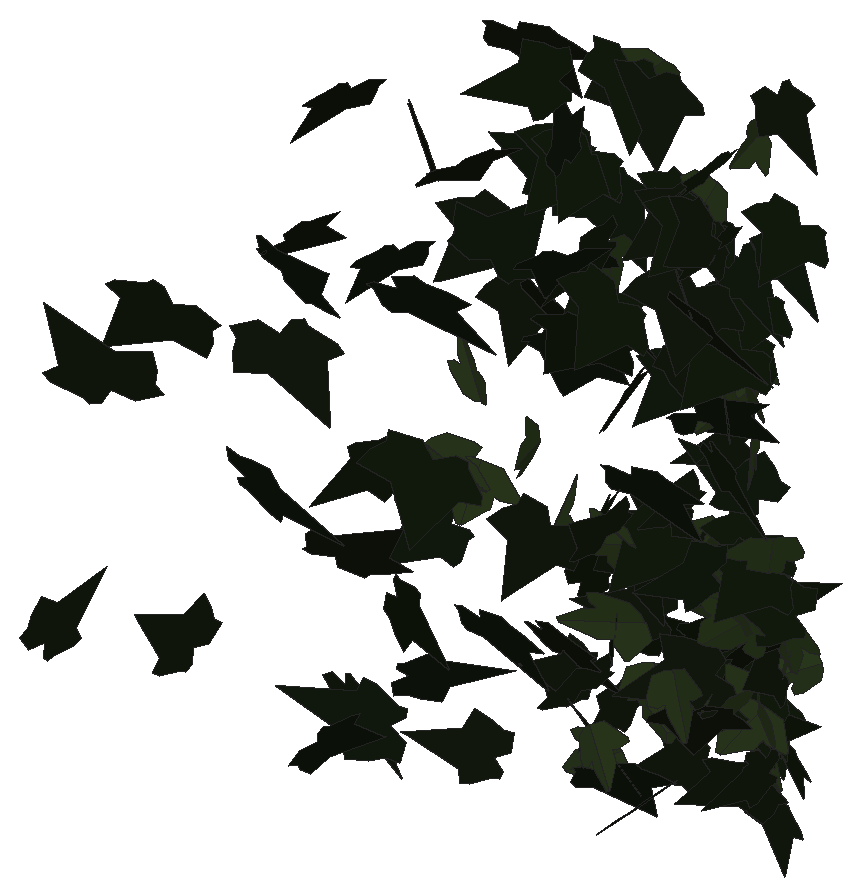
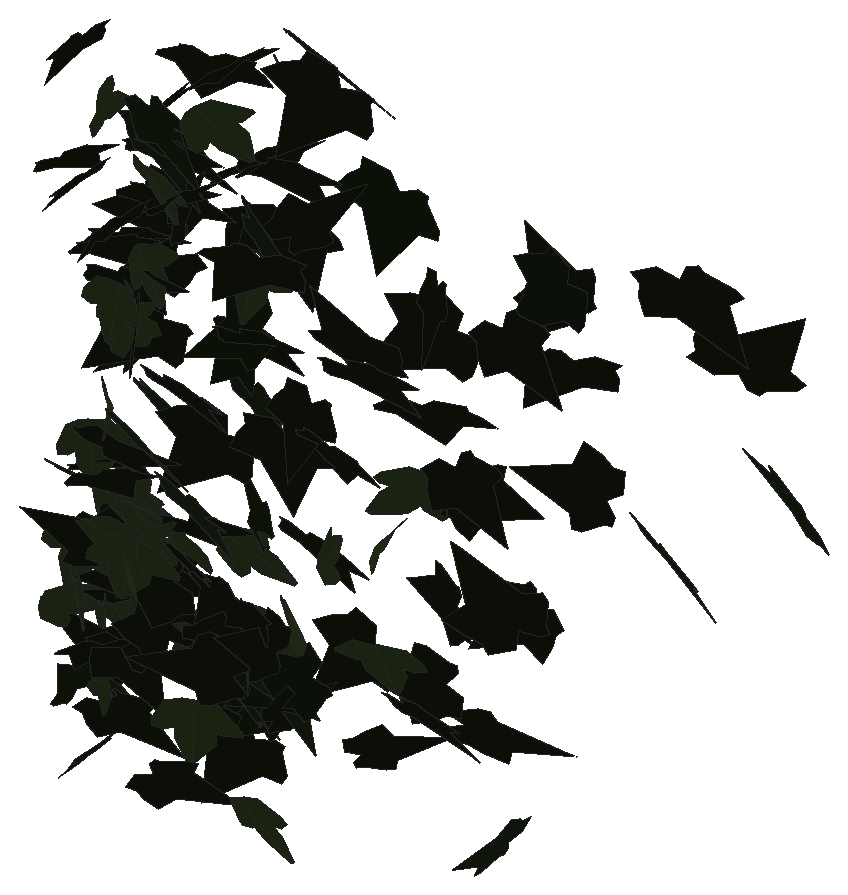
# SketchUp Ruby script. Lengths in inches.
U = 1.inch
M = Sketchup.active_model
def pt(a) = Geom::Point3d.new(a.map { |v| v * U })
def face(e, loops, mat)
  f = e.add_face(loops[0].map { |a| pt(a) })
  loops[1..].each { |l| e.add_face(l.map { |a| pt(a) }).erase! }
  f.material = f.back_material = mat if mat
  f
end
# faces: each face lists its corners as indices into pts; further lists are holes
def faces(e, pts, list, mat = nil) = list.each { |f| face(e, (f[0].is_a?(Array) ? f : [f]).map { |l| l.map { |i| pts[i] } }, mat) }
# xy, xz, yz: faces in a plane at the given z, y or x. An outline is a flat list of corners, or four numbers for a rectangle; further outlines are holes
def ring(l) = l.size == 4 ? [[l[0], l[1]], [l[2], l[1]], [l[2], l[3]], [l[0], l[3]]] : l.each_slice(2).to_a
def flat(e, list, mat, &to3) = list.each { |f| face(e, (f[0].is_a?(Array) ? f : [f]).map { |l| ring(l).map { |u, v| to3.(u, v) } }, mat) }
def xy(e, z, list, mat = nil) = flat(e, list, mat) { |x, y| [x, y, z] }
def xz(e, y, list, mat = nil) = flat(e, list, mat) { |x, z| [x, y, z] }
def yz(e, x, list, mat = nil) = flat(e, list, mat) { |y, z| [x, y, z] }
def lines(e, pts, list) = list.each { |a, b| e.add_line(pt(pts[a]), pt(pts[b])) }
# prism: a flat outline (further loops are holes) pulled along v
def prism(e, loops, v, mat = nil)
  f = face(e, loops, mat); d = Geom::Vector3d.new(v.map { |x| x * U })
  f.pushpull(f.normal.samedirection?(d) ? d.length : -d.length)
end
def box(e, o, s, mat = nil) = prism(e, [[o, [o[0] + s[0], o[1], o[2]], [o[0] + s[0], o[1] + s[1], o[2]], [o[0], o[1] + s[1], o[2]]]], [0, 0, s[2]], mat)
def at(x, y, z, deg = 0) = Geom::Transformation.translation(pt([x, y, z])) * Geom::Transformation.rotation(ORIGIN, Z_AXIS, deg.degrees)
def axes(o, x, y, z) = Geom::Transformation.new([*x, 0, *y, 0, *z, 0, *pt(o).to_a, 1])
def part(name) = M.definitions.add(name)
# library, detail: a bought-in or finely detailed component or shape, given as its bounding box
def library(name, o, s) = part(name).tap { |d| box(d.entities, o, s) }
def detail(e, o, s) = box(e.add_group.entities, o, s)
def put(e, d, t, mat = nil) = e.add_instance(d, t).tap { |i| i.material = mat if mat }
def group(e, t, mat = nil) = e.add_group.tap { |g| g.transformation = t; g.material = mat if mat }.entities
root = M.entities
M.materials.add("1026 AP 7946 SUNNY SIDE UP").color = [254, 231, 186]
M.materials.add("efeu1").color = [18, 25, 13]
M.materials.add("efeu2").color = [43, 57, 29]
c1 = part("ivyleaf_9")
p = [[1.54,2.16,1.25],[1.36,2.04,1.19],[-0.21,0.99,0.68],[-0.71,1.11,0.82],[-0.85,0.86,0.67],[-0.8,0.17,0.21],
  [-0.9,-0.01,0.1],[-0.67,-0.16,-0.02],[-0.08,-0.08,-0.05],[-0.03,-0.6,-0.4],[0.65,-0.88,-0.66],[0.83,-0.6,-0.49],
  [1.29,-0.42,-0.43],[1.8125,-0.07,-0.26],[1.21,0.44,0.15]]
faces(c1.entities,p,[[0,1,2,3,4,5,6,7,8,9,10,11,12,13,14]],"efeu1")
c2 = part("ivyleaf_10")
p = [[0,0.5,-0.03],[-0.0625,2.02,-0.43],[-0.19,2.01,-0.46],[-0.54,1.05,-0.29],[-0.52,0.625,-0.18],[-0.83,0.76,-0.28],
  [-1.16,0.64,-0.33],[-1.15,0.33,-0.24],[-0.77,-0.39,0.02],[-0.3,-0.51,0.16],[0.04,-0.48,0.23],[-0.02,2.01,-0.4375],
  [-0.06,2.01,-0.43],[0.04,-0.49,0.23],[0.67,-0.49,0.14],[1.38,0.36,-0.2],[1.375,0.51,-0.24],[0.81,0.65,-0.19],
  [0.62,0.59,-0.15],[0.6,1.09,-0.28],[0.5,1.23,-0.31]]
faces(c2.entities,p,[[0,1,2,3,4,5,6,7,8,9,10],[11,12,0,13,14,15,16,17,18,19,20]],"efeu2")
put(root,c1,axes([90.28,204.37,282.83],[-0.24358,0.38021,0.10952],[0.06838,-0.08884,0.43377],[0.66272,0.14891,-0.0045]),"1026 AP 7946 SUNNY SIDE UP")
put(root,c1,axes([90.01,206.08,285.99],[0.29721,0.05151,0.38408],[-0.60755,0.0827,0.17576],[-0.08959,-0.38992,0.08224]),"1026 AP 7946 SUNNY SIDE UP")
put(root,c1,axes([91.6,205.9,282.51],[-0.23197,0.30623,0.25862],[-0.19167,0.20953,-0.35575],[-0.6294,-0.17667,0.01302]),"1026 AP 7946 SUNNY SIDE UP")
put(root,c1,axes([90.74,206.5,287.33],[0.23481,0.09165,-0.38264],[-0.42428,-0.25925,-0.17776],[-0.46344,0.28377,-0.03114]),"1026 AP 7946 SUNNY SIDE UP")
put(root,c1,axes([93.29,206.64,281.26],[-0.08853,0.12697,-0.37628],[-0.15546,0.34144,0.15068],[0.61777,0.10412,-0.01601]),"1026 AP 7946 SUNNY SIDE UP")
put(root,c1,axes([91.22,207.6875,284.22],[0.40642,-0.15866,0.28639],[0.33268,-0.1885,-0.30774],[0.41385,0.30734,-0.03386]),"1026 AP 7946 SUNNY SIDE UP")
put(root,c1,axes([91.49,208.1,287.43],[0.57582,-0.10896,-0.15139],[0.2568,0.0199,0.37613],[-0.15728,-0.36642,0.05986]),"1026 AP 7946 SUNNY SIDE UP")
put(root,c1,axes([91.51,208.01,286.4375],[-0.16156,-0.27217,-0.28485],[0.1869,0.23904,-0.30471],[0.61412,-0.14435,0.0178]),"1026 AP 7946 SUNNY SIDE UP")
put(root,c1,axes([93.84,208.41,285.09],[-0.48199,-0.26527,-0.10385],[0.16958,0.02915,-0.41271],[0.44635,-0.29752,0.04466]),"1026 AP 7946 SUNNY SIDE UP")
put(root,c1,axes([91.42,208.27,287.83],[0.25122,0.26891,0.23765],[0.2212,0.17693,-0.32517],[-0.54497,0.19577,-0.02244]),"1026 AP 7946 SUNNY SIDE UP")
put(root,c1,axes([92.78,208.71,280.45],[-0.32348,-0.12983,-0.30399],[-0.39375,-0.16084,0.2446],[-0.35087,0.30019,0.00576]),"1026 AP 7946 SUNNY SIDE UP")
put(root,c1,axes([92.92,208.85,282.4],[0.09531,-0.09706,-0.3787],[0.61631,-0.02708,0.06952],[-0.07289,-0.35589,0.09263]),"1026 AP 7946 SUNNY SIDE UP")
put(root,c1,axes([96.6,209.03,288.3],[-0.25614,-0.32528,0.20811],[-0.10783,-0.18919,-0.38597],[0.63794,-0.16258,0.01832]),"1026 AP 7946 SUNNY SIDE UP")
put(root,c1,axes([92.53,209.01,284.44],[-0.10498,0.00796,-0.395],[0.14058,-0.36437,-0.02835],[-0.61067,-0.08525,0.06138]),"1026 AP 7946 SUNNY SIDE UP")
put(root,c1,axes([91.69,209.06,282.58],[0.59044,0.15415,-0.01146],[-0.0079,0.04169,0.40563],[0.26245,-0.34555,0.03798]),"1026 AP 7946 SUNNY SIDE UP")
put(root,c1,axes([96.49,208.91,284.66],[-0.14634,0.32567,0.15798],[-0.08423,0.13502,-0.35854],[-0.5981,-0.0987,0.01184]),"1026 AP 7946 SUNNY SIDE UP")
put(root,c1,axes([96.03,209.13,287.6],[0.27288,0.13159,-0.30791],[-0.34397,-0.20738,-0.22439],[-0.41571,0.25797,-0.01645]),"1026 AP 7946 SUNNY SIDE UP")
put(root,c1,axes([93.04,209.01,281.18],[0.18415,0.2178,-0.27133],[0.10731,0.25128,0.26078],[0.56076,-0.11961,0.0392]),"1026 AP 7946 SUNNY SIDE UP")
put(root,c1,axes([92.68,209.21,287.05],[0.6573,0.06501,0.09122],[0.15221,-0.02734,-0.41843],[-0.09756,0.39534,-0.03825]),"1026 AP 7946 SUNNY SIDE UP")
put(root,c1,axes([93.95,209.57,279.99],[-0.17113,-0.01295,0.33509],[-0.4862,-0.12982,-0.10626],[0.21613,-0.3023,0.02628]),"1026 AP 7946 SUNNY SIDE UP")
put(root,c2,axes([95.96,209.375,281.05],[0.07273,0.33107,0.01199],[0.01082,0.00611,-0.35726],[-0.56202,0.04296,-0.00533]),"1026 AP 7946 SUNNY SIDE UP")
put(root,c2,axes([97.1875,209.54,282.27],[0.4331,-0.08334,0.22855],[0.32153,-0.10601,-0.28667],[0.22204,0.31606,-0.03068]),"1026 AP 7946 SUNNY SIDE UP")
put(root,c1,axes([97.93,209.42,284.3125],[-0.45991,0.24915,0.02602],[-0.06086,-0.00798,-0.39284],[-0.42007,-0.27162,0.02842]),"1026 AP 7946 SUNNY SIDE UP")
put(root,c1,axes([96.71,209.28,280.24],[0.03469,0.37547,0.12003],[0.01979,0.10673,-0.40104],[-0.66257,0.02285,-0.0057]),"1026 AP 7946 SUNNY SIDE UP")
put(root,c2,axes([93.08,209.46,284.55],[-0.34261,-0.15364,-0.24766],[0.37491,0.08055,-0.26473],[0.28111,-0.29468,0.05122]),"1026 AP 7946 SUNNY SIDE UP")
put(root,c1,axes([95.04,209.62,291.03],[-0.54914,0.19561,0.07717],[-0.13967,-0.00261,-0.40199],[-0.32355,-0.33087,0.04256]),"1026 AP 7946 SUNNY SIDE UP")
put(root,c1,axes([97.42,210.05,289.23],[-0.17996,-0.19101,0.31705],[-0.17291,-0.28215,-0.23585],[0.5764,-0.14428,0.02824]),"1026 AP 7946 SUNNY SIDE UP")
put(root,c1,axes([95.3125,209.51,290.01],[0.00313,0.11265,0.39841],[-0.04172,0.36997,-0.11508],[-0.65633,-0.02298,0.00922]),"1026 AP 7946 SUNNY SIDE UP")
put(root,c1,axes([93.41,209.53,289.15],[0.2412,0.37899,0.09819],[0.03464,0.08499,-0.43199],[-0.65909,0.14316,0.01323]),"1026 AP 7946 SUNNY SIDE UP")
put(root,c1,axes([97.4375,209.69,281.83],[0.30649,0.26126,-0.1198],[-0.08848,-0.10398,-0.34105],[-0.47663,0.1873,-0.01372]),"1026 AP 7946 SUNNY SIDE UP")
put(root,c1,axes([93.67,209.79,281.92],[0.63362,-0.01268,-0.04615],[-0.0746,-0.03474,-0.39845],[0.01454,0.37411,-0.03329]),"1026 AP 7946 SUNNY SIDE UP")
put(root,c1,axes([95.12,209.8,288.19],[0.16397,0.32864,-0.15217],[-0.07703,-0.13927,-0.36864],[-0.60588,0.10665,0.00569]),"1026 AP 7946 SUNNY SIDE UP")
put(root,c1,axes([97.47,210.02,282.3],[-0.60196,0.06601,0.09509],[-0.15787,-0.02152,-0.38441],[-0.09963,-0.36472,0.03462]),"1026 AP 7946 SUNNY SIDE UP")
put(root,c1,axes([97.02,210.04,287.83],[0.44864,-0.16709,0.1738],[0.20653,-0.11421,-0.335],[0.34029,0.2896,-0.02582]),"1026 AP 7946 SUNNY SIDE UP")
put(root,c1,axes([91.03,210.08,279.79],[0.30427,-0.33021,-0.03507],[-0.01877,0.02637,-0.40186],[0.5623,0.17956,0.00556]),"1026 AP 7946 SUNNY SIDE UP")
put(root,c1,axes([94.49,210.16,283.52],[-0.59937,-0.03075,-0.15291],[0.24537,-0.02672,-0.37781],[0.03126,-0.37979,0.0336]),"1026 AP 7946 SUNNY SIDE UP")
put(root,c1,axes([97.04,210.21,288.15],[-0.48786,-0.2239,-0.13843],[0.20303,0.05137,-0.38788],[0.38636,-0.30972,0.02904]),"1026 AP 7946 SUNNY SIDE UP")
put(root,c1,axes([97.47,210.14,285.68],[0.36619,-0.27433,-0.05768],[-0.08023,0.02671,-0.3726],[0.4666,0.21989,-0.0188]),"1026 AP 7946 SUNNY SIDE UP")
put(root,c2,axes([97.75,210.35,282.01],[0.00476,-0.02498,0.3479],[0.03758,-0.32454,-0.03142],[0.55255,0.02229,-0.00086]),"1026 AP 7946 SUNNY SIDE UP")
put(root,c1,axes([95.03,210.39,289.49],[-0.24032,-0.31552,0.1567],[-0.05092,-0.1508,-0.3708],[0.59123,-0.14124,0.03176]),"1026 AP 7946 SUNNY SIDE UP")
put(root,c1,axes([97.69,210.35,287.37],[-0.50073,-0.20031,0.03423],[-0.01264,-0.05026,-0.38034],[0.34484,-0.29271,0.03576]),"1026 AP 7946 SUNNY SIDE UP")
put(root,c1,axes([95.42,210.24,288.3],[-0.4811,0.20682,-0.20993],[0.22752,-0.1516,-0.37554],[-0.43054,-0.31121,0.03613]),"1026 AP 7946 SUNNY SIDE UP")
put(root,c1,axes([97.09,210.4,289.13],[-0.41864,-0.21772,0.09656],[-0.08882,-0.0809,-0.3523],[0.39199,-0.25086,0.0233]),"1026 AP 7946 SUNNY SIDE UP")
put(root,c1,axes([97.49,210.0625,289],[-0.25637,0.33466,0.03547],[-0.06393,0.01448,-0.3917],[-0.5666,-0.15306,0.02814]),"1026 AP 7946 SUNNY SIDE UP")
put(root,c1,axes([95.04,210.2,280.72],[0.51109,-0.19488,-0.05836],[-0.09684,0.00728,-0.38295],[0.3284,0.30544,-0.0221]),"1026 AP 7946 SUNNY SIDE UP")
put(root,c2,axes([97.79,210.27,283.1],[-0.44981,0.00742,0.22798],[-0.35369,-0.07947,-0.27583],[0.07495,-0.33046,0.06657]),"1026 AP 7946 SUNNY SIDE UP")
put(root,c1,axes([95.92,209.97,286.09],[-0.16185,0.14812,-0.34149],[-0.33688,0.2526,0.19147],[0.49648,0.21969,0.0186]),"1026 AP 7946 SUNNY SIDE UP")
put(root,c1,axes([94.94,210.47,289.48],[-0.58601,-0.15376,-0.00557],[0.02315,-0.02278,-0.40391],[0.26004,-0.34447,0.0234]),"1026 AP 7946 SUNNY SIDE UP")
put(root,c1,axes([96.84,210.46,289.13],[-0.57945,-0.04375,0.01249],[-0.01272,-0.03722,-0.36693],[0.07606,-0.33953,0.03374]),"1026 AP 7946 SUNNY SIDE UP")
put(root,c2,axes([97.67,210.27,283.27],[-0.22751,0.04524,0.32245],[-0.50905,0.03417,-0.14817],[-0.08459,-0.32735,0.02439]),"1026 AP 7946 SUNNY SIDE UP")
put(root,c1,axes([95.09,210.41,283.54],[0.03299,0.24718,0.22068],[-0.07855,-0.19897,0.26145],[0.53715,-0.04428,0.02468]),"1026 AP 7946 SUNNY SIDE UP")
put(root,c1,axes([95.47,210.24,279.95],[0.48475,0.21422,0.00873],[0.03169,-0.01598,-0.38153],[-0.36237,0.28516,-0.02169]),"1026 AP 7946 SUNNY SIDE UP")
put(root,c1,axes([97.87,210.68,283.78],[-0.38029,-0.22783,0.12324],[-0.03763,-0.13899,-0.33404],[0.43398,-0.21169,0.07903]),"1026 AP 7946 SUNNY SIDE UP")
put(root,c1,axes([96.72,210.39,287.94],[0.06571,-0.26019,0.28328],[0.01202,0.26989,0.2832],[-0.63396,-0.02185,0.03473]),"1026 AP 7946 SUNNY SIDE UP")
put(root,c1,axes([95.52,210.66,290.96],[-0.09479,-0.38255,0.04381],[-0.01928,-0.04473,-0.41449],[0.65377,-0.05678,-0.00587]),"1026 AP 7946 SUNNY SIDE UP")
put(root,c1,axes([95.95,210.5625,290.9],[-0.38038,-0.23962,-0.19924],[0.2509,0.1114,-0.3484],[0.44607,-0.26699,0.02607]),"1026 AP 7946 SUNNY SIDE UP")
put(root,c1,axes([95.9,210.33,284.73],[0.636,0.07083,-0.02131],[-0.02333,-0.03897,-0.40696],[-0.12313,0.37321,-0.033]),"1026 AP 7946 SUNNY SIDE UP")
put(root,c1,axes([96.9,210.23,287.22],[0.12884,-0.06857,-0.39529],[-0.0414,0.37412,-0.07472],[0.63466,0.03832,0.07538]),"1026 AP 7946 SUNNY SIDE UP")
put(root,c2,axes([97.84,210.52,281.57],[0.53443,-0.00012,-0.12716],[-0.20044,-0.03686,-0.33553],[-0.0219,0.33446,-0.0323]),"1026 AP 7946 SUNNY SIDE UP")
put(root,c1,axes([95.51,210.59,280.94],[-0.42379,0.10851,-0.15282],[0.19254,-0.09703,-0.28982],[-0.23822,-0.27146,0.03763]),"1026 AP 7946 SUNNY SIDE UP")
put(root,c1,axes([93.85,210.36,291.03],[0.64688,0.13183,-0.03746],[-0.0355,-0.05125,-0.43012],[-0.22958,0.37939,-0.03905]),"1026 AP 7946 SUNNY SIDE UP")
put(root,c1,axes([94.94,210.3,281.07],[-0.08285,0.3329,0.16237],[-0.16864,0.13082,-0.34988],[-0.59452,-0.0835,0.07662]),"1026 AP 7946 SUNNY SIDE UP")
put(root,c1,axes([97.08,210.3,286.18],[0.46367,0.23296,0.15629],[0.21748,0.0694,-0.38217],[-0.40985,0.30037,-0.02598]),"1026 AP 7946 SUNNY SIDE UP")
put(root,c1,axes([98.45,210.57,283.36],[-0.46259,0.19403,0.17398],[-0.34123,-0.02631,-0.33277],[-0.25652,-0.3149,0.12892]),"1026 AP 7946 SUNNY SIDE UP")
put(root,c1,axes([97.92,210.59,282.76],[-0.12561,0.25885,-0.2124],[0.09297,-0.1942,-0.29093],[-0.54933,-0.09205,-0.00067]),"1026 AP 7946 SUNNY SIDE UP")
put(root,c2,axes([96.08,210.57,281.54],[0.48944,0.15768,0.08279],[0.11157,0.03672,-0.3513],[-0.27482,0.29571,0.00483]),"1026 AP 7946 SUNNY SIDE UP")
put(root,c1,axes([94.55,210.82,280.89],[-0.0861,-0.02396,0.33079],[-0.36902,-0.22084,-0.05956],[0.37569,-0.22241,0.01731]),"1026 AP 7946 SUNNY SIDE UP")
put(root,c1,axes([94.18,210.57,281.55],[0.59779,-0.1006,0.05024],[0.07478,-0.02136,-0.39228],[0.17401,0.35479,-0.004]),"1026 AP 7946 SUNNY SIDE UP")
put(root,c2,axes([97.29,210.86,286.28],[-0.13332,-0.16887,0.3042],[-0.03788,-0.29089,-0.19427],[0.56304,-0.05956,0.05896]),"1026 AP 7946 SUNNY SIDE UP")
put(root,c1,axes([94.22,210.85,288.8],[0.0102,0.03385,0.40828],[-0.53482,-0.2155,0.02281],[0.36796,-0.31416,0.02184]),"1026 AP 7946 SUNNY SIDE UP")
put(root,c2,axes([97.96,210.55,281.68],[-0.3177,0.24151,0.14085],[-0.22659,0.05516,-0.31858],[-0.40527,-0.22016,0.06771]),"1026 AP 7946 SUNNY SIDE UP")
put(root,c1,axes([97.3125,210.52,286.51],[0.21423,-0.11273,-0.32609],[-0.46065,0.1401,-0.17477],[0.29866,0.29695,-0.03567]),"1026 AP 7946 SUNNY SIDE UP")
put(root,c2,axes([95.35,210.6875,283.34],[-0.21009,0.00149,0.31271],[-0.47311,-0.09551,-0.12724],[0.14834,-0.3025,0.03708]),"1026 AP 7946 SUNNY SIDE UP")
put(root,c1,axes([97.58,210.89,281.92],[-0.40636,-0.24477,0.07764],[-0.04849,-0.07748,-0.36591],[0.43223,-0.23881,0.03195]),"1026 AP 7946 SUNNY SIDE UP")
put(root,c2,axes([95.44,210.71,282.12],[0.23959,-0.01756,-0.33345],[-0.52894,0.00224,-0.15138],[0.01577,0.34174,-0.01136]),"1026 AP 7946 SUNNY SIDE UP")
put(root,c2,axes([97.99,210.7,284.21],[-0.35209,-0.28172,-0.00173],[0.02655,-0.01407,-0.37405],[0.47751,-0.20695,0.01952]),"1026 AP 7946 SUNNY SIDE UP")
put(root,c1,axes([97.9,210.71,280.6],[-0.44246,0.21451,-0.08069],[0.07266,-0.07061,-0.36126],[-0.3807,-0.26279,0.02483]),"1026 AP 7946 SUNNY SIDE UP")
put(root,c1,axes([93.12,210.66,287.125],[-0.36144,0.1392,0.29242],[0.39364,-0.141,0.27029],[0.33619,0.31475,-0.0021]),"1026 AP 7946 SUNNY SIDE UP")
put(root,c1,axes([96,210.92,283.57],[-0.51502,-0.16394,0.0249],[-0.01319,-0.03884,-0.3683],[0.2813,-0.30197,0.02832]),"1026 AP 7946 SUNNY SIDE UP")
put(root,c1,axes([97.85,211,282.12],[-0.09535,-0.13666,0.30515],[-0.15775,-0.27146,-0.16174],[0.51574,-0.1083,0.00694]),"1026 AP 7946 SUNNY SIDE UP")
put(root,c1,axes([96.91,210.67,289.75],[-0.24105,0.33904,-0.04648],[-0.00004,-0.0518,-0.39366],[-0.58123,-0.1406,0.0193]),"1026 AP 7946 SUNNY SIDE UP")
put(root,c1,axes([97.27,210.93,287.13],[-0.52112,-0.18198,-0.03314],[0.05902,-0.00269,-0.3815],[0.30708,-0.3083,0.01708]),"1026 AP 7946 SUNNY SIDE UP")
put(root,c2,axes([95.05,210.73,287.86],[-0.2473,-0.30358,-0.10204],[0.09342,0.07479,-0.359],[0.52999,-0.15484,0.01567]),"1026 AP 7946 SUNNY SIDE UP")
put(root,c2,axes([97.375,210.54,286.72],[-0.06801,0.10121,0.35448],[-0.26572,0.29053,-0.11176],[-0.52185,-0.16112,0.01071]),"1026 AP 7946 SUNNY SIDE UP")
put(root,c1,axes([94.89,210.8,287.02],[0.55199,-0.19306,0.01499],[0.01047,-0.02194,-0.40481],[0.32876,0.32485,-0.01228]),"1026 AP 7946 SUNNY SIDE UP")
put(root,c1,axes([91.78,210.7,288.68],[0.35222,-0.11981,-0.29579],[-0.4402,0.09579,-0.25305],[0.25513,0.33068,-0.02826]),"1026 AP 7946 SUNNY SIDE UP")
put(root,c1,axes([96.5,210.84,281.53],[0.38576,0.2209,0.12595],[-0.16777,-0.06256,0.33755],[0.38784,-0.24678,0.02074]),"1026 AP 7946 SUNNY SIDE UP")
put(root,c2,axes([96.83,210.9375,287.53],[-0.06355,-0.332,0.05563],[-0.00224,-0.05649,-0.35843],[0.57162,-0.03713,0.00478]),"1026 AP 7946 SUNNY SIDE UP")
put(root,c1,axes([97.41,210.98,280.17],[0.04705,0.02081,-0.32588],[-0.29167,-0.25184,-0.03867],[-0.42856,0.17368,-0.00946]),"1026 AP 7946 SUNNY SIDE UP")
put(root,c1,axes([94.96,211.05,287],[-0.53122,-0.10048,0.00793],[0.00216,-0.03236,-0.35073],[0.1712,-0.31138,0.02905]),"1026 AP 7946 SUNNY SIDE UP")
put(root,c1,axes([90.34,210.95,288.63],[-0.11816,0.27777,-0.25916],[0.04535,-0.24559,-0.30876],[-0.62788,-0.07001,0.02647]),"1026 AP 7946 SUNNY SIDE UP")
put(root,c1,axes([96.17,211.2,288.79],[-0.2895,-0.2235,0.21221],[-0.13824,-0.18826,-0.30051],[0.49134,-0.18466,0.04049]),"1026 AP 7946 SUNNY SIDE UP")
put(root,c2,axes([97.55,210.79,286.56],[-0.30079,0.20639,0.19721],[-0.24426,0.11435,-0.28798],[-0.39753,-0.22643,0.02773]),"1026 AP 7946 SUNNY SIDE UP")
put(root,c1,axes([94.84,211.12,281.5625],[0.01188,0.09647,0.36514],[-0.0687,-0.33742,0.09873],[0.59569,-0.04084,0.00411]),"1026 AP 7946 SUNNY SIDE UP")
put(root,c1,axes([96.58,210.69,282.32],[0.08773,0.21836,-0.2991],[0.08756,0.2776,0.24393],[0.59938,-0.07252,0.00814]),"1026 AP 7946 SUNNY SIDE UP")
put(root,c2,axes([93.37,211.2,283.97],[0.00766,0.03634,0.3541],[0.23719,-0.2999,0.0291],[0.51177,0.13845,-0.01878]),"1026 AP 7946 SUNNY SIDE UP")
put(root,c1,axes([97.36,211.16,287.7],[-0.31122,-0.26991,0.022],[0.00379,-0.03056,-0.34915],[0.45999,-0.18237,0.01776]),"1026 AP 7946 SUNNY SIDE UP")
put(root,c2,axes([97.08,210.97,282.78],[-0.27372,0.2733,-0.03821],[0.00991,-0.04207,-0.33985],[-0.46859,-0.16053,0.01513]),"1026 AP 7946 SUNNY SIDE UP")
put(root,c1,axes([97.43,211.19,283.95],[-0.35653,-0.24883,0.02743],[-0.00186,-0.03675,-0.34826],[0.42523,-0.20879,0.02147]),"1026 AP 7946 SUNNY SIDE UP")
put(root,c1,axes([92.9,211.2,287.26],[-0.6114,-0.0963,0.00108],[0.00925,-0.02911,-0.39828],[0.16326,-0.35899,0.0266]),"1026 AP 7946 SUNNY SIDE UP")
put(root,c1,axes([97.15,211.09,280.98],[0.04408,0.02293,0.366],[0.45104,-0.21735,-0.00903],[0.36644,0.26477,-0.0329]),"1026 AP 7946 SUNNY SIDE UP")
put(root,c1,axes([97.11,211.04,281.27],[0.02372,0.26478,-0.20744],[-0.0439,-0.1959,-0.28629],[-0.55873,0.02663,0.01369]),"1026 AP 7946 SUNNY SIDE UP")
put(root,c2,axes([97.41,211.21,280.65],[-0.22416,0.08648,-0.28191],[0.23182,-0.2349,-0.15852],[-0.41151,-0.17943,0.06426]),"1026 AP 7946 SUNNY SIDE UP")
put(root,c1,axes([95.52,211.29,282.02],[-0.19457,-0.03827,0.32072],[-0.44915,-0.14288,-0.12969],[0.24894,-0.2877,0.01667]),"1026 AP 7946 SUNNY SIDE UP")
put(root,c1,axes([91.04,211.14,286.24],[-0.06465,0.2806,-0.24239],[0.03082,-0.22957,-0.30617],[-0.61519,-0.04099,0.01013]),"1026 AP 7946 SUNNY SIDE UP")
put(root,c1,axes([91.875,211.21,282.19],[-0.58201,0.03311,-0.01575],[0.01974,-0.03632,-0.36736],[-0.05857,-0.34126,0.0327]),"1026 AP 7946 SUNNY SIDE UP")
put(root,c2,axes([96.49,211.18,289.09],[0.49031,-0.18649,-0.02447],[-0.05802,-0.01544,-0.36674],[0.31314,0.28914,-0.02964]),"1026 AP 7946 SUNNY SIDE UP")
put(root,c1,axes([97.94,211.37,288.97],[-0.27876,-0.28305,0.10909],[-0.06439,-0.10101,-0.34416],[0.47171,-0.18106,0.01748]),"1026 AP 7946 SUNNY SIDE UP")
put(root,c2,axes([97.24,211.1,286.87],[-0.51215,0.14785,0.02271],[-0.05198,-0.01884,-0.35849],[-0.2477,-0.30173,0.02828]),"1026 AP 7946 SUNNY SIDE UP")
put(root,c1,axes([97.73,211.18,288.67],[0.15435,-0.28928,-0.12849],[-0.05021,0.11254,-0.32302],[0.52685,0.09548,0.00686]),"1026 AP 7946 SUNNY SIDE UP")
put(root,c1,axes([97.08,211.18,288.19],[0.15511,-0.32127,-0.15697],[-0.0742,0.13564,-0.35566],[0.59193,0.10119,-0.00345]),"1026 AP 7946 SUNNY SIDE UP")
put(root,c2,axes([97.83,211.16,282.73],[-0.53958,0.10205,-0.01781],[0.01441,-0.03213,-0.3566],[-0.17531,-0.31674,0.0255]),"1026 AP 7946 SUNNY SIDE UP")
put(root,c1,axes([97.3125,211.28,281.29],[-0.11303,-0.2962,-0.13624],[0.09716,0.11304,-0.32197],[0.53596,-0.08296,0.02963]),"1026 AP 7946 SUNNY SIDE UP")
put(root,c1,axes([96.02,211.01,283.99],[-0.13599,0.29604,0.18477],[-0.20484,0.13745,-0.3176],[-0.54096,-0.12647,0.07382]),"1026 AP 7946 SUNNY SIDE UP")
put(root,c2,axes([97.15,211.4,285.26],[-0.13364,0.16495,-0.27904],[0.03323,-0.26794,-0.19007],[-0.52565,-0.05888,0.05893]),"1026 AP 7946 SUNNY SIDE UP")
put(root,c1,axes([96.07,211.36,286.01],[-0.56828,-0.00333,-0.07823],[0.12364,-0.0447,-0.35587],[-0.0107,-0.33971,0.04277]),"1026 AP 7946 SUNNY SIDE UP")
put(root,c2,axes([97.18,211.48,290.07],[0.05108,0.08604,-0.35183],[-0.10794,-0.32381,-0.10118],[-0.56835,0.06923,-0.01241]),"1026 AP 7946 SUNNY SIDE UP")
put(root,c2,axes([94.69,211.23,279.55],[0.38857,-0.1411,-0.21765],[-0.31403,0.08261,-0.28581],[0.27518,0.29353,-0.01882]),"1026 AP 7946 SUNNY SIDE UP")
put(root,c1,axes([94.53,211.28,288.48],[-0.21185,-0.2273,-0.28806],[0.24216,0.22494,-0.27419],[0.54249,-0.18917,0.0099]),"1026 AP 7946 SUNNY SIDE UP")
put(root,c1,axes([97.6875,211.28,290.9375],[0.12722,-0.2981,-0.18084],[-0.10007,0.16261,-0.31682],[0.53332,0.10162,-0.01631]),"1026 AP 7946 SUNNY SIDE UP")
put(root,c2,axes([95.6875,211.28,280.77],[-0.51865,-0.15918,0.0052],[0.01596,-0.03297,-0.36753],[0.26999,-0.30382,0.03171]),"1026 AP 7946 SUNNY SIDE UP")
put(root,c1,axes([97.625,211.48,280.6],[0.06323,-0.22935,0.19811],[0.07152,-0.1835,-0.25111],[0.49836,0.05543,0.0109]),"1026 AP 7946 SUNNY SIDE UP")
put(root,c1,axes([94.07,211.22,285.76],[0.4108,0.1432,-0.22318],[-0.27833,-0.13422,-0.30166],[-0.33033,0.29118,-0.02338]),"1026 AP 7946 SUNNY SIDE UP")
put(root,c1,axes([93.67,211.18,286.37],[0.4987,-0.03045,-0.23716],[-0.37413,0.01837,-0.31592],[0.06006,0.36724,0.00131]),"1026 AP 7946 SUNNY SIDE UP")
put(root,c1,axes([97.44,211.47,279.55],[0.03281,-0.30601,0.08378],[0.00678,-0.08296,-0.31647],[0.49854,0.02126,-0.00121]),"1026 AP 7946 SUNNY SIDE UP")
put(root,c1,axes([94.875,211.37,282.92],[-0.24385,-0.07991,-0.33573],[0.51038,0.09089,-0.17154],[0.19855,-0.33176,0.02862]),"1026 AP 7946 SUNNY SIDE UP")
put(root,c2,axes([95.3,211.45,290.53],[-0.29223,-0.19105,0.24584],[-0.20695,-0.20015,-0.27594],[0.4665,-0.20847,0.03159]),"1026 AP 7946 SUNNY SIDE UP")
put(root,c2,axes([92.39,211.15,284.58],[-0.00748,0.28694,-0.20969],[-0.13347,0.1937,0.30265],[0.57815,0.04843,0.06716]),"1026 AP 7946 SUNNY SIDE UP")
put(root,c2,axes([97.28,211.36,283.22],[0.40601,-0.02481,-0.21944],[-0.34809,0.00365,-0.25698],[0.03604,0.31476,-0.0099]),"1026 AP 7946 SUNNY SIDE UP")
put(root,c1,axes([97.28,211.21,282.83],[0.00864,0.0202,0.35484],[0.55951,0.03776,-0.00736],[-0.06473,0.32906,-0.01627]),"1026 AP 7946 SUNNY SIDE UP")
put(root,c2,axes([96.54,211.58,282.56],[0.00153,-0.02625,-0.34644],[0.13641,-0.31316,0.0231],[-0.53338,-0.08017,0.00492]),"1026 AP 7946 SUNNY SIDE UP")
put(root,c1,axes([97.24,211.29,284.5],[-0.10077,0.13336,0.3025],[-0.45007,0.12756,-0.12307],[-0.27556,-0.25712,0.0904]),"1026 AP 7946 SUNNY SIDE UP")
put(root,c2,axes([92.2,211.43,283.03],[0.56829,0.0851,-0.04271],[-0.04986,-0.04973,-0.36792],[-0.15241,0.33359,-0.03889]),"1026 AP 7946 SUNNY SIDE UP")
put(root,c2,axes([96.22,211.6,283.41],[-0.04544,-0.19623,0.26812],[0.06336,-0.26254,-0.2],[0.51001,0.01513,0.04873]),"1026 AP 7946 SUNNY SIDE UP")
put(root,c2,axes([97.92,211.6,281.9],[-0.11564,-0.01452,0.31123],[-0.11097,-0.29037,-0.03595],[0.48182,-0.07036,0.06642]),"1026 AP 7946 SUNNY SIDE UP")
put(root,c1,axes([95.9,211.49,283.45],[-0.47915,0.05752,-0.10067],[0.14434,-0.04095,-0.31889],[-0.10542,-0.31748,0.02094]),"1026 AP 7946 SUNNY SIDE UP")
put(root,c1,axes([96.08,211.58,279.76],[-0.04503,-0.05311,-0.32586],[-0.16821,-0.28717,0.05902],[-0.49558,0.1023,0.00957]),"1026 AP 7946 SUNNY SIDE UP")
put(root,c2,axes([97.74,211.35,282.26],[0.2215,-0.25821,-0.15241],[-0.06156,0.14455,-0.30046],[0.46271,0.14284,0.03298]),"1026 AP 7946 SUNNY SIDE UP")
put(root,c1,axes([93.01,211.57,286.11],[-0.45582,-0.07503,-0.19961],[0.32835,-0.01798,-0.29226],[0.08683,-0.32585,0.05729]),"1026 AP 7946 SUNNY SIDE UP")
put(root,c2,axes([96.67,211.4375,283.1],[-0.5463,-0.13624,-0.03856],[0.0943,-0.04481,-0.36871],[0.21904,-0.32052,0.06257]),"1026 AP 7946 SUNNY SIDE UP")
put(root,c1,axes([94.3125,211.19,282.2],[0.01923,0.03108,0.36266],[0.39871,0.2439,-0.029],[-0.41677,0.23477,-0.01101]),"1026 AP 7946 SUNNY SIDE UP")
put(root,c2,axes([93.7,211.41,282.79],[0.28233,-0.26968,0.07075],[-0.03428,0.06918,0.33958],[-0.47155,-0.16649,0.01767]),"1026 AP 7946 SUNNY SIDE UP")
put(root,c1,axes([95.03,211.3,281.625],[0.26351,0.06228,0.32686],[0.51594,0.04076,-0.17423],[-0.11034,0.33935,-0.0341]),"1026 AP 7946 SUNNY SIDE UP")
put(root,c1,axes([96.85,211.46,285.12],[-0.43573,0.20437,0.01542],[-0.04243,-0.01261,-0.35038],[-0.34491,-0.25664,0.02363]),"1026 AP 7946 SUNNY SIDE UP")
